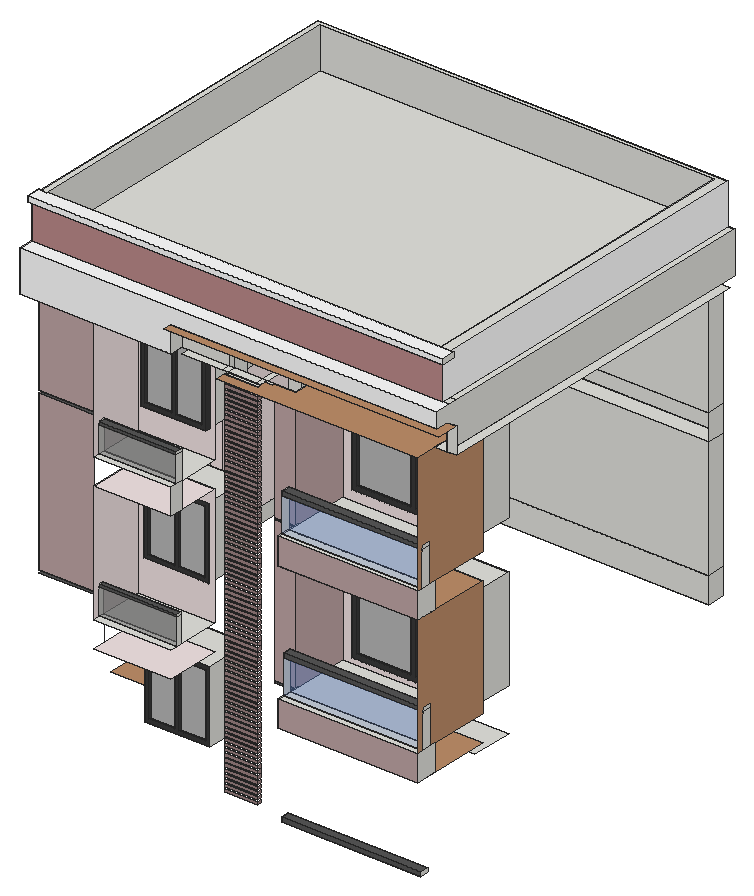
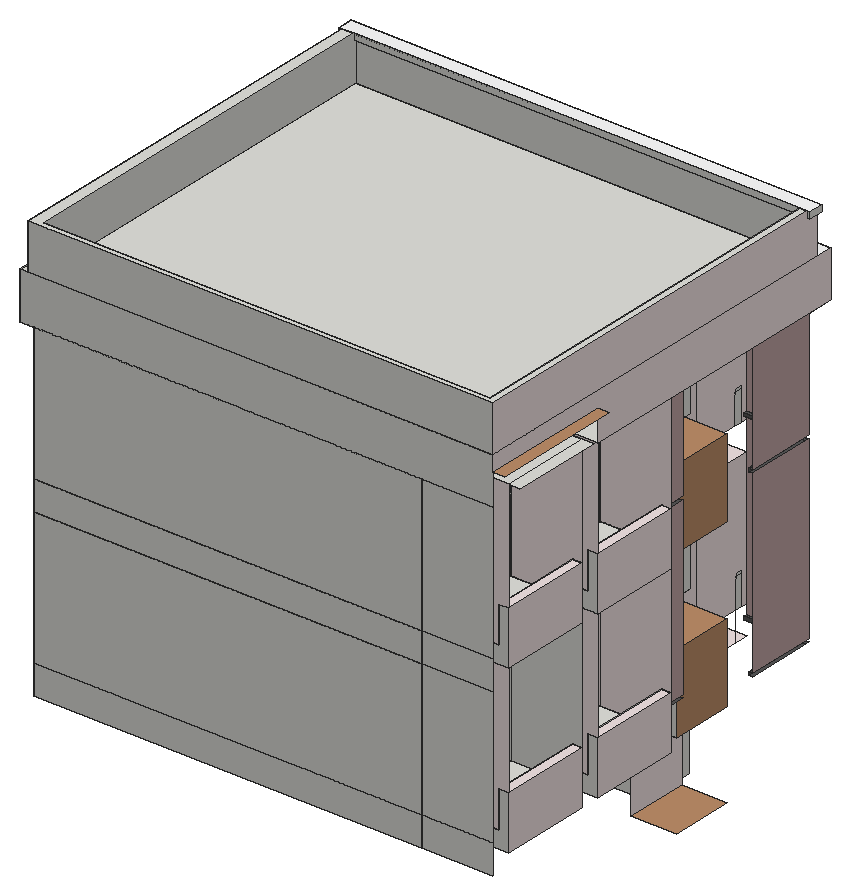
# SketchUp Ruby script. Lengths in inches.
U = 1.inch
M = Sketchup.active_model
def pt(a) = Geom::Point3d.new(a.map { |v| v * U })
def face(e, loops, mat)
  f = e.add_face(loops[0].map { |a| pt(a) })
  loops[1..].each { |l| e.add_face(l.map { |a| pt(a) }).erase! }
  f.material = f.back_material = mat if mat
  f
end
# faces: each face lists its corners as indices into pts; further lists are holes
def faces(e, pts, list, mat = nil) = list.each { |f| face(e, (f[0].is_a?(Array) ? f : [f]).map { |l| l.map { |i| pts[i] } }, mat) }
# xy, xz, yz: faces in a plane at the given z, y or x. An outline is a flat list of corners, or four numbers for a rectangle; further outlines are holes
def ring(l) = l.size == 4 ? [[l[0], l[1]], [l[2], l[1]], [l[2], l[3]], [l[0], l[3]]] : l.each_slice(2).to_a
def flat(e, list, mat, &to3) = list.each { |f| face(e, (f[0].is_a?(Array) ? f : [f]).map { |l| ring(l).map { |u, v| to3.(u, v) } }, mat) }
def xy(e, z, list, mat = nil) = flat(e, list, mat) { |x, y| [x, y, z] }
def xz(e, y, list, mat = nil) = flat(e, list, mat) { |x, z| [x, y, z] }
def yz(e, x, list, mat = nil) = flat(e, list, mat) { |y, z| [x, y, z] }
def lines(e, pts, list) = list.each { |a, b| e.add_line(pt(pts[a]), pt(pts[b])) }
# prism: a flat outline (further loops are holes) pulled along v
def prism(e, loops, v, mat = nil)
  f = face(e, loops, mat); d = Geom::Vector3d.new(v.map { |x| x * U })
  f.pushpull(f.normal.samedirection?(d) ? d.length : -d.length)
end
def box(e, o, s, mat = nil) = prism(e, [[o, [o[0] + s[0], o[1], o[2]], [o[0] + s[0], o[1] + s[1], o[2]], [o[0], o[1] + s[1], o[2]]]], [0, 0, s[2]], mat)
def at(x, y, z, deg = 0) = Geom::Transformation.translation(pt([x, y, z])) * Geom::Transformation.rotation(ORIGIN, Z_AXIS, deg.degrees)
def axes(o, x, y, z) = Geom::Transformation.new([*x, 0, *y, 0, *z, 0, *pt(o).to_a, 1])
def part(name) = M.definitions.add(name)
# library, detail: a bought-in or finely detailed component or shape, given as its bounding box
def library(name, o, s) = part(name).tap { |d| box(d.entities, o, s) }
def detail(e, o, s) = box(e.add_group.entities, o, s)
def put(e, d, t, mat = nil) = e.add_instance(d, t).tap { |i| i.material = mat if mat }
def group(e, t, mat = nil) = e.add_group.tap { |g| g.transformation = t; g.material = mat if mat }.entities
root = M.entities
M.materials.add("Generic").color = [188, 139, 139]
M.materials.add("Generic\#1").color = [192, 166, 166]
M.materials.add("Generic\#2").color = [190, 142, 105]
M.materials.add("Generic\#3").color = [158, 131, 131]
M.materials.add("Generic\#4").color = [242, 228, 228]
M.materials.add("[Color M00]").color = [255, 255, 255]
M.materials.add("[Color M06]").color = [86, 86, 86]
M.materials.add("[Color M07]").color = [58, 58, 58]
M.materials.add("[Mirror 01]").color = [183, 183, 183]
M.materials.add("[Translucent Glass Blue]").color = [98, 147, 234]
M.materials["[Translucent Glass Blue]"].alpha = 0.21
M.materials.add("[Translucent Glass Gray]").color = [128, 128, 128]
M.materials["[Translucent Glass Gray]"].alpha = 0.5
c1 = part("Group\#1")
xy(c1.entities,0,[[0,0,90.75,6]],"[Color M07]")
xy(c1.entities,5.41,[[5.41,0,42.67,3],[48.08,0,85.34,3]],"[Color M07]")
xy(c1.entities,95.34,[[5.41,0,42.67,3],[48.08,0,85.34,3]],"[Color M07]")
xy(c1.entities,100.75,[[0,0,90.75,6]],"[Color M07]")
xz(c1.entities,0,[[[0,0,90.75,100.75],[48.08,5.41,85.34,95.34],[5.41,5.41,42.67,95.34]]],"[Color M07]")
xz(c1.entities,3,[[5.41,5.41,42.67,95.34],[48.08,5.41,85.34,95.34]],"[Mirror 01]")
xz(c1.entities,6,[[0,0,90.75,100.75]],"[Mirror 01]")
yz(c1.entities,0,[[0,0,6,100.75]],"[Color M07]")
yz(c1.entities,5.41,[[0,5.41,3,95.34]],"[Color M07]")
yz(c1.entities,42.67,[[0,5.41,3,95.34]],"[Color M07]")
yz(c1.entities,48.08,[[0,5.41,3,95.34]],"[Color M07]")
yz(c1.entities,85.34,[[0,5.41,3,95.34]],"[Color M07]")
yz(c1.entities,90.75,[[0,0,6,100.75]],"[Color M07]")
c2 = part("Group\#3")
xy(c2.entities,0,[[0,0,45.875,5.125]])
xz(c2.entities,0,[[0,0,45.875,4.1875]])
yz(c2.entities,45.875,[[0,0,5.125,4.1875]])
c3 = part("Group\#2")
xy(c3.entities,0,[[0,0,173,6]],"[Color M07]")
xy(c3.entities,7.67,[[90.33,0,165.33,3]],"[Color M06]")
xy(c3.entities,7.67,[[7.67,0,82.67,3]],"[Color M07]")
xy(c3.entities,134.58,[[7.67,0,82.67,3],[90.33,0,165.33,3]],"[Color M07]")
xy(c3.entities,142.25,[[0,0,173,6]],"[Color M07]")
xz(c3.entities,0,[[[0,0,173,142.25],[7.67,7.67,82.67,134.58],[90.33,7.67,165.33,134.58]]],"[Color M07]")
xz(c3.entities,3,[[7.67,7.67,82.67,134.58],[90.33,7.67,165.33,134.58]],"[Mirror 01]")
xz(c3.entities,6,[[0,0,173,142.25]],"[Mirror 01]")
yz(c3.entities,0,[[0,0,6,142.25]],"[Color M07]")
yz(c3.entities,7.67,[[0,7.67,3,134.58]],"[Color M07]")
yz(c3.entities,82.67,[[0,7.67,3,134.58]],"[Color M07]")
yz(c3.entities,90.33,[[0,7.67,3,134.58]],"[Color M07]")
yz(c3.entities,165.33,[[0,7.67,3,134.58]],"[Color M07]")
yz(c3.entities,173,[[0,0,6,142.25]],"[Color M07]")
xy(root,455.21,[[162.5,105,253.25,171.75]])
xy(root,457.125,[[421.3125,20.9,617.3125,32.9]])
xy(root,462.9375,[[421.3125,20.9,617.3125,32.9]],"[Color M06]")
xy(root,470.25,[[80.75,147.9375,137.3125,225.85]],"Generic\#2")
xy(root,555.96,[[162.5,105,253.25,171.75]])
xy(root,559.68,[[434.09,128.4375,607.09,187.0625]])
xy(root,577.125,[[137.3125,525.6875,145.6875,549.6875],[145.6875,525.6875,617.3125,549.6875]])
xy(root,577.125,[[421.3125,15.0625,617.3125,128.4375],[80.75,147.9375,137.3125,225.85]],"Generic\#2")
xy(root,577.125,[[152.75,27.5625,261.3125,105]],"Generic\#4")
xy(root,592.1875,[[49.25,273.85,137.3125,387.77],[49.25,411.77,137.3125,525.6875]],"Generic\#4")
xy(root,610.6875,[[392.6875,45.6875,421.3125,50.375]],"[Color M06]")
xy(root,613.6875,[[421.3125,15.0625,617.3125,24.5],[421.3125,24.5,617.3125,36.5],[152.75,27.5625,261.3125,37.125],[421.3125,36.5,617.3125,128.4375],[152.75,37.125,261.3125,44.125],
  [152.75,44.125,261.3125,105],[61.25,273.85,137.3125,387.77],[61.25,411.77,137.3125,525.6875],[137.3125,525.6875,145.6875,549.6875],[145.6875,525.6875,617.3125,549.6875]])
xy(root,613.6875,[[392.6875,45.6875,421.3125,50.375]],"[Color M06]")
xy(root,620.55,[[434.09,128.4375,607.09,187.0625]])
xy(root,621.63,[[49.25,61.3125,126.1875,66],[49.25,66,53.9375,147.9375]],"[Color M06]")
xy(root,623.77,[[73.1875,225.85,77.875,249.85]],"[Color M06]")
xy(root,625.63,[[49.25,61.3125,126.1875,66],[49.25,66,53.9375,147.9375]],"[Color M06]")
xy(root,627.77,[[73.1875,225.85,77.875,249.85]],"[Color M06]")
xy(root,650.625,[[152.75,37.125,261.3125,44.125]])
xy(root,654.1875,[[152.75,37.125,261.3125,44.125]],"[Color M06]")
xy(root,658.8125,[[49.25,273.85,61.25,387.77],[49.25,411.77,61.25,525.6875]],"Generic\#4")
xy(root,660.15,[[161.5625,105,252.3125,171.75]])
xy(root,661.6875,[[421.3125,24.5,617.3125,36.5]])
xy(root,667.5,[[421.3125,24.5,617.3125,36.5]],"[Color M06]")
xy(root,674.8125,[[80.75,147.9375,137.3125,225.85]],"Generic\#2")
xy(root,760.9,[[161.5625,105,252.3125,171.75]])
xy(root,762.8,[[434.09,128.4375,607.09,187.0625]])
xy(root,781.6875,[[137.3125,525.6875,617.3125,549.6875]])
xy(root,781.6875,[[421.3125,15.0625,617.3125,128.4375],[80.75,147.9375,137.3125,225.85]],"Generic\#2")
xy(root,781.6875,[[152.75,27.5625,261.3125,105]],"Generic\#4")
xy(root,796.75,[[49.25,273.85,137.3125,387.77],[49.25,411.77,137.3125,525.6875]],"Generic\#4")
xy(root,815.25,[[392.6875,45.6875,421.3125,50.375]],"[Color M06]")
xy(root,818.25,[[421.3125,15.0625,617.3125,22.5625],[421.3125,22.5625,617.3125,34.5625],[152.75,27.5625,261.3125,36.375],[421.3125,34.5625,617.3125,128.4375],[152.75,36.375,261.3125,45.6875],
  [152.75,45.6875,261.3125,105],[61.25,273.85,137.3125,387.77],[61.25,411.77,137.3125,525.6875],[137.3125,525.6875,617.3125,549.6875]])
xy(root,818.25,[[392.6875,45.6875,421.3125,50.375]],"[Color M06]")
xy(root,831.74,[[434.09,128.4375,607.09,187.0625]])
xy(root,843.44,[[73.1875,225.85,77.875,249.85]],"[Color M06]")
xy(root,847.32,[[49.25,61.3125,126.1875,66],[49.25,66,53.9375,147.9375]],"[Color M06]")
xy(root,847.44,[[73.1875,225.85,77.875,249.85]],"[Color M06]")
xy(root,851.32,[[49.25,61.3125,126.1875,66],[49.25,66,53.9375,147.9375]],"[Color M06]")
xy(root,854.96,[[161.8125,105,252.5625,171.75]])
xy(root,855.1875,[[152.75,36.375,261.3125,45.6875]])
xy(root,858.75,[[152.75,36.375,261.3125,45.6875]],"[Color M06]")
xy(root,863.375,[[49.25,273.85,61.25,387.77],[49.25,411.77,61.25,525.6875]],"Generic\#4")
xy(root,866.25,[[421.3125,22.5625,617.3125,34.5625]])
xy(root,872.0625,[[421.3125,22.5625,617.3125,34.5625]],"[Color M06]")
xy(root,879.375,[[80.75,147.9375,137.3125,225.85]],"Generic\#2")
xy(root,955.71,[[161.8125,105,252.5625,171.75]])
xy(root,973.99,[[434.09,128.4375,607.09,187.0625]])
xy(root,986.25,[[49.25,27.5625,126.1875,61.3125],[126.1875,27.5625,152.75,45.6875],[152.75,27.5625,261.3125,105],[336,28.6875,381.875,33.8125],[271.74,33.8125,328.375,45.6875],
  [328.375,33.8125,336,45.6875],[336,33.8125,375.18,45.6875],[375.18,33.8125,381.875,45.6875],[381.875,41.875,392.6875,45.6875],[375.18,45.6875,381.875,157.1],
  [617.3125,45.6875,634.3125,128.4375],[634.3125,45.6875,647.125,525.6875],[617.3125,128.4375,634.3125,525.6875],[49.25,147.9375,49.25,249.85,73.1875,249.85,73.1875,225.85,137.3125,225.85,137.3125,147.9375],[73.1875,225.85,137.3125,249.85],
  [49.25,249.85,137.3125,273.85],[49.25,273.85,137.3125,387.77],[137.3125,525.6875,617.3125,549.6875],[617.3125,525.6875,634.3125,549.6875]])
xy(root,986.25,[[336,15.0625,336,28.6875,381.875,28.6875,381.875,41.875,392.6875,41.875,392.6875,45.6875,421.3125,45.6875,421.3125,128.4375,617.3125,128.4375,617.3125,15.0625]],"Generic\#2")
xy(root,1000.9375,[[34.875,411.77,49.25,525.6875],[49.25,411.77,137.3125,525.6875]])
xy(root,1022.8125,[[261.3125,27.5625,634.3125,45.6875]])
xy(root,1022.8125,[[261.3125,15.0625,647.125,15.0625,647.125,45.6875,634.3125,45.6875,634.3125,27.5625,261.3125,27.5625]],"Generic\#2")
xy(root,1024.8125,[[34.875,387.77,49.25,549.6875]],"Generic\#2")
xy(root,1044.4375,[[[49.25,48.6875,624.9375,549.6875],[58.0625,60.6875,609.9375,543.0625]],[624.9375,48.6875,634.3125,60.6875],[58.0625,60.6875,609.9375,543.0625],[624.9375,60.6875,634.3125,549.6875]])
xy(root,1044.4375,[[49.25,27.5625,634.3125,48.6875]],"[Color M00]")
xy(root,1093.625,[[45.75,45.1875,628.4375,48.6875],[45.75,48.6875,49.25,64.1875],[49.25,48.6875,49.25,64.1875,58.0625,64.1875,58.0625,60.6875,624.9375,60.6875,624.9375,48.6875],[624.9375,48.6875,628.4375,60.6875],[58.0625,60.6875,609.9375,64.1875],
  [609.9375,60.6875,624.9375,64.1875],[624.9375,60.6875,628.4375,64.1875]])
xy(root,1101.375,[[49.25,64.1875,58.0625,64.1875,58.0625,543.0625,609.9375,543.0625,609.9375,64.1875,624.9375,64.1875,624.9375,549.6875,49.25,549.6875]])
xy(root,1101.375,[[45.75,45.1875,628.4375,64.1875]],"[Color M00]")
xz(root,15.0625,[[421.3125,577.125,617.3125,613.6875],[421.3125,781.6875,617.3125,818.25]],"Generic\#1")
xz(root,20.9,[[421.3125,457.125,617.3125,462.9375]],"[Color M06]")
xz(root,22.5625,[[421.3125,866.25,617.3125,872.0625]],"[Color M06]")
xz(root,22.5625,[[421.3125,818.25,617.3125,866.25]],"[Translucent Glass Blue]")
xz(root,24.5,[[421.3125,661.6875,617.3125,667.5]],"[Color M06]")
xz(root,24.5,[[421.3125,613.6875,617.3125,661.6875]],"[Translucent Glass Blue]")
xz(root,27.5625,[[49.25,986.25,261.3125,986.25,261.3125,1022.8125,634.3125,1022.8125,634.3125,1044.4375,49.25,1044.4375]],"[Color M00]")
xz(root,32.9,[[421.3125,457.125,617.3125,462.9375]])
xz(root,33.8125,[[336,982.0625,375.18,986.25],[375.18,982.0625,381.875,986.25]])
xz(root,34.5625,[[421.3125,866.25,617.3125,872.0625]])
xz(root,34.5625,[[421.3125,818.25,617.3125,866.25]],"[Translucent Glass Blue]")
xz(root,36.375,[[152.75,855.1875,261.3125,858.75]],"[Color M06]")
xz(root,36.375,[[152.75,818.25,261.3125,855.1875]],"[Translucent Glass Gray]")
xz(root,36.5,[[421.3125,661.6875,617.3125,667.5]])
xz(root,36.5,[[421.3125,613.6875,617.3125,661.6875]],"[Translucent Glass Blue]")
xz(root,37.125,[[152.75,650.625,261.3125,654.1875]],"[Color M06]")
xz(root,37.125,[[152.75,613.6875,261.3125,650.625]],"[Translucent Glass Gray]")
xz(root,44.125,[[152.75,650.625,261.3125,654.1875]])
xz(root,44.125,[[152.75,613.6875,261.3125,650.625]],"[Translucent Glass Gray]")
xz(root,45.1875,[[45.75,1093.625,628.4375,1101.375]],"[Color M00]")
xz(root,45.6875,[[152.75,855.1875,261.3125,858.75],[261.3125,986.25,328.375,1022.8125],[634.3125,986.25,647.125,1022.8125]])
xz(root,45.6875,[[392.6875,613.6875,421.3125,815.25],[392.6875,818.25,421.3125,986.25]],"Generic\#1")
xz(root,45.6875,[[152.75,818.25,261.3125,855.1875]],"[Translucent Glass Gray]")
xz(root,48.6875,[[49.25,1044.4375,624.9375,1093.625]],"Generic")
xz(root,50.375,[[392.6875,610.6875,421.3125,613.6875],[392.6875,815.25,421.3125,818.25]],"[Color M06]")
xz(root,60.6875,[[58.0625,1044.4375,609.9375,1093.625]])
xz(root,61.3125,[[49.25,625.63,126.1875,847.32],[49.25,851.32,126.1875,986.25]],"Generic\#1")
xz(root,64.1875,[[45.75,1093.625,49.25,1101.375],[49.25,1093.625,58.0625,1101.375],[58.0625,1093.625,609.9375,1101.375],[609.9375,1093.625,624.9375,1101.375],[624.9375,1093.625,628.4375,1101.375]])
xz(root,66,[[53.9375,621.63,126.1875,625.63],[53.9375,847.32,126.1875,851.32]],"[Color M06]")
xz(root,105,[[[152.75,613.6875,261.3125,781.6875],[161.5625,660.15,252.3125,760.9]],[[152.75,818.25,261.3125,986.25],[161.8125,854.96,252.5625,955.71]]],"Generic\#4")
xz(root,128.4375,[[[421.3125,613.6875,617.3125,781.6875],[434.09,620.55,607.09,762.8]],[[421.3125,818.25,617.3125,986.25],[434.09,831.74,607.09,973.99]]],"Generic\#4")
xz(root,171.75,[[162.5,455.21,253.25,555.96],[161.5625,660.15,252.3125,760.9],[161.8125,854.96,252.5625,955.71]])
xz(root,187.0625,[[434.09,620.55,607.09,762.8],[434.09,831.74,607.09,973.99]])
xz(root,225.85,[[80.75,577.125,137.3125,674.8125],[80.75,781.6875,137.3125,879.375]])
xz(root,249.85,[[73.1875,577.125,137.3125,613.6875],[73.1875,613.6875,137.3125,613.6875,137.3125,781.6875,73.1875,781.6875,73.1875,627.77,77.875,627.77,77.875,623.77,73.1875,623.77],[73.1875,781.6875,137.3125,818.25],[73.1875,818.25,137.3125,818.25,137.3125,986.25,73.1875,986.25,73.1875,847.44,77.875,847.44,77.875,843.44,73.1875,843.44]])
xz(root,273.85,[[49.25,592.1875,49.25,658.8125,61.25,658.8125,61.25,613.6875,137.3125,613.6875,137.3125,592.1875],[49.25,796.75,49.25,863.375,61.25,863.375,61.25,818.25,137.3125,818.25,137.3125,796.75]])
xz(root,273.85,[[61.25,613.6875,61.25,658.8125,49.25,658.8125,49.25,796.75,137.3125,796.75,137.3125,613.6875],[61.25,818.25,61.25,863.375,49.25,863.375,49.25,986.25,137.3125,986.25,137.3125,818.25]],"Generic\#4")
xz(root,387.77,[[49.25,592.1875,137.3125,592.1875,137.3125,613.6875,61.25,613.6875,61.25,658.8125,49.25,658.8125],[49.25,796.75,137.3125,796.75,137.3125,818.25,61.25,818.25,61.25,863.375,49.25,863.375]])
xz(root,387.77,[[61.25,613.6875,137.3125,613.6875,137.3125,796.75,49.25,796.75,49.25,658.8125,61.25,658.8125],[61.25,818.25,137.3125,818.25,137.3125,986.25,49.25,986.25,49.25,863.375,61.25,863.375]],"Generic\#4")
xz(root,411.77,[[49.25,592.1875,49.25,658.8125,61.25,658.8125,61.25,613.6875,137.3125,613.6875,137.3125,592.1875],[61.25,613.6875,61.25,658.8125,49.25,658.8125,49.25,796.75,137.3125,796.75,137.3125,613.6875],[49.25,796.75,49.25,863.375,61.25,863.375,61.25,818.25,137.3125,818.25,137.3125,796.75]])
xz(root,411.77,[[61.25,818.25,61.25,863.375,49.25,863.375,49.25,1000.9375,137.3125,1000.9375,137.3125,818.25]],"Generic\#4")
xz(root,525.6875,[[137.3125,577.125,145.6875,613.6875],[145.6875,577.125,617.3125,613.6875],[49.25,592.1875,137.3125,592.1875,137.3125,613.6875,61.25,613.6875,61.25,658.8125,49.25,658.8125],[137.3125,613.6875,617.3125,781.6875],[49.25,796.75,137.3125,796.75,137.3125,818.25,61.25,818.25,61.25,863.375,49.25,863.375],
  [137.3125,818.25,617.3125,986.25]])
xz(root,525.6875,[[61.25,613.6875,137.3125,613.6875,137.3125,796.75,49.25,796.75,49.25,658.8125,61.25,658.8125],[61.25,818.25,137.3125,818.25,137.3125,1000.9375,49.25,1000.9375,49.25,863.375,61.25,863.375]],"Generic\#4")
xz(root,543.0625,[[58.0625,1044.4375,609.9375,1101.375]])
xz(root,549.6875,[[49.25,577.125,137.3125,613.6875],[137.3125,577.125,617.3125,613.6875],[49.25,613.6875,137.3125,781.6875],[137.3125,613.6875,617.3125,781.6875],[49.25,781.6875,137.3125,818.25],
  [137.3125,781.6875,617.3125,818.25],[49.25,818.25,137.3125,986.25],[137.3125,818.25,617.3125,986.25],[49.25,986.25,634.3125,1044.4375],[49.25,1044.4375,624.9375,1101.375]])
yz(root,45.75,[[45.1875,1093.625,64.1875,1101.375]])
yz(root,49.25,[[61.3125,625.63,147.9375,847.32],[61.3125,851.32,147.9375,986.25]],"Generic\#1")
yz(root,49.25,[[273.85,592.1875,387.77,658.8125],[411.77,592.1875,525.6875,658.8125],[273.85,796.75,387.77,863.375],[411.77,796.75,525.6875,863.375],[27.5625,986.25,27.5625,1044.4375,549.6875,1044.4375,549.6875,1024.8125,387.77,1024.8125,387.77,986.25],
  [48.6875,1044.4375,48.6875,1093.625,64.1875,1093.625,64.1875,1101.375,549.6875,1101.375,549.6875,1044.4375]],"Generic\#4")
yz(root,53.9375,[[66,621.63,147.9375,625.63],[66,847.32,147.9375,851.32]],"[Color M06]")
yz(root,58.0625,[[60.6875,1044.4375,543.0625,1044.4375,543.0625,1101.375,64.1875,1101.375,64.1875,1093.625,60.6875,1093.625]])
yz(root,61.25,[[273.85,613.6875,387.77,658.8125],[411.77,613.6875,525.6875,658.8125],[273.85,818.25,387.77,863.375],[411.77,818.25,525.6875,863.375]])
yz(root,73.1875,[[225.85,627.77,249.85,843.44],[225.85,847.44,249.85,986.25]],"Generic\#1")
yz(root,77.875,[[225.85,623.77,249.85,627.77],[225.85,843.44,249.85,847.44]],"[Color M06]")
yz(root,80.75,[[147.9375,577.125,225.85,674.8125],[147.9375,781.6875,225.85,879.375]],"Generic\#2")
yz(root,137.3125,[[157.1,577.125,225.85,674.8125],[525.6875,577.125,549.6875,613.6875],[273.85,592.1875,387.77,613.6875],[411.77,592.1875,525.6875,613.6875],[411.77,613.6875,525.6875,796.75],
  [525.6875,613.6875,549.6875,781.6875],[157.1,781.6875,225.85,796.75],[525.6875,781.6875,549.6875,818.25],[157.1,796.75,225.85,879.375],[225.85,796.75,249.85,986.25],
  [249.85,796.75,273.85,986.25],[273.85,796.75,387.77,818.25],[387.77,796.75,411.77,986.25],[411.77,796.75,525.6875,818.25],[273.85,818.25,387.77,986.25],
  [411.77,818.25,525.6875,986.25],[525.6875,818.25,549.6875,986.25]])
yz(root,137.3125,[[147.9375,470.25,225.85,577.125],[273.85,613.6875,387.77,796.75],[147.9375,674.8125,225.85,781.6875],[147.9375,879.375,225.85,986.25],[411.77,986.25,525.6875,1000.9375]],"Generic\#4")
yz(root,152.75,[[37.125,613.6875,44.125,650.625],[37.125,650.625,44.125,654.1875],[36.375,818.25,45.6875,855.1875],[36.375,855.1875,45.6875,858.75]])
yz(root,152.75,[[27.5625,613.6875,37.125,613.6875,37.125,654.1875,44.125,654.1875,44.125,613.6875,105,613.6875,105,781.6875,27.5625,781.6875],[27.5625,818.25,36.375,818.25,36.375,858.75,45.6875,858.75,45.6875,818.25,105,818.25,105,986.25,27.5625,986.25]],"Generic\#4")
yz(root,161.5625,[[105,660.15,171.75,760.9]])
yz(root,161.8125,[[105,854.96,171.75,955.71]])
yz(root,162.5,[[105,455.21,171.75,555.96]])
yz(root,252.3125,[[105,660.15,171.75,760.9]])
yz(root,252.5625,[[105,854.96,171.75,955.71]])
yz(root,253.25,[[105,455.21,171.75,555.96]])
yz(root,261.3125,[[37.125,613.6875,44.125,650.625],[37.125,650.625,44.125,654.1875],[27.5625,781.6875,45.6875,818.25],[36.375,818.25,45.6875,855.1875],[36.375,855.1875,45.6875,858.75],
  [27.5625,986.25,45.6875,1022.8125]])
yz(root,336,[[28.6875,982.0625,33.8125,986.25]])
yz(root,392.6875,[[45.6875,610.6875,50.375,613.6875],[45.6875,815.25,50.375,818.25]],"[Color M06]")
yz(root,421.3125,[[20.9,457.125,32.9,462.9375],[15.0625,577.125,15.0625,613.6875,50.375,613.6875,50.375,610.6875,45.6875,610.6875,45.6875,577.125],[24.5,613.6875,36.5,661.6875],[24.5,661.6875,36.5,667.5],[15.0625,781.6875,15.0625,818.25,50.375,818.25,50.375,815.25,45.6875,815.25,45.6875,781.6875],
  [22.5625,818.25,34.5625,866.25],[22.5625,866.25,34.5625,872.0625]])
yz(root,421.3125,[[45.6875,613.6875,128.4375,781.6875],[45.6875,818.25,128.4375,986.25]],"Generic\#1")
yz(root,434.09,[[128.4375,620.55,187.0625,762.8],[128.4375,831.74,187.0625,973.99]])
yz(root,607.09,[[128.4375,620.55,187.0625,762.8],[128.4375,831.74,187.0625,973.99]])
yz(root,609.9375,[[60.6875,1044.4375,60.6875,1093.625,64.1875,1093.625,64.1875,1101.375,543.0625,1101.375,543.0625,1044.4375]])
yz(root,617.3125,[[20.9,457.125,32.9,462.9375],[15.0625,577.125,45.6875,613.6875],[525.6875,577.125,549.6875,613.6875],[24.5,613.6875,36.5,661.6875],[525.6875,613.6875,549.6875,781.6875],
  [24.5,661.6875,36.5,667.5],[15.0625,781.6875,45.6875,818.25],[525.6875,781.6875,549.6875,818.25],[22.5625,818.25,34.5625,866.25],[525.6875,818.25,549.6875,986.25],
  [22.5625,866.25,34.5625,872.0625]])
yz(root,617.3125,[[15.0625,613.6875,15.0625,781.6875,128.4375,781.6875,128.4375,613.6875,36.5,613.6875,36.5,667.5,24.5,667.5,24.5,613.6875],[15.0625,818.25,15.0625,986.25,128.4375,986.25,128.4375,818.25,34.5625,818.25,34.5625,872.0625,22.5625,872.0625,22.5625,818.25]],"Generic\#2")
yz(root,624.9375,[[48.6875,1044.4375,549.6875,1044.4375,549.6875,1101.375,64.1875,1101.375,64.1875,1093.625,48.6875,1093.625]],"[Color M00]")
yz(root,628.4375,[[45.1875,1093.625,64.1875,1101.375]])
yz(root,634.3125,[[45.6875,986.25,549.6875,986.25,549.6875,1044.4375,27.5625,1044.4375,27.5625,1022.8125,45.6875,1022.8125]])
p = [[336,45.6875,986.25],[336,45.6875,1022.8125],[152.75,45.6875,613.6875],[152.75,45.6875,577.125],[271.74,157.1,986.25],[137.3125,157.1,986.25]]
lines(root,p,[[0,1],[2,3],[4,5]])
put(root,c1,at(162.5,105,455.21))
put(root,c2,at(336,28.6875,460.625),"Generic\#3")
put(root,c2,at(336,28.6875,467.0625),"Generic\#3")
put(root,c2,at(336,28.6875,473.5),"Generic\#3")
put(root,c2,at(336,28.6875,479.9375),"Generic\#3")
put(root,c2,at(336,28.6875,486.375),"Generic\#3")
put(root,c2,at(336,28.6875,492.8125),"Generic\#3")
put(root,c2,at(336,28.6875,499.25),"Generic\#3")
put(root,c2,at(336,28.6875,505.6875),"Generic\#3")
put(root,c2,at(336,28.6875,512.125),"Generic\#3")
put(root,c2,at(336,28.6875,518.5625),"Generic\#3")
put(root,c2,at(336,28.6875,525),"Generic\#3")
put(root,c2,at(336,28.6875,531.4375),"Generic\#3")
put(root,c2,at(336,28.6875,537.875),"Generic\#3")
put(root,c2,at(336,28.6875,544.3125),"Generic\#3")
put(root,c2,at(336,28.6875,550.75),"Generic\#3")
put(root,c2,at(336,28.6875,557.1875),"Generic\#3")
put(root,c2,at(336,28.6875,563.625),"Generic\#3")
put(root,c2,at(336,28.6875,570.0625),"Generic\#3")
put(root,c2,at(336,28.6875,576.5),"Generic\#3")
put(root,c2,at(336,28.6875,582.9375),"Generic\#3")
put(root,c2,at(336,28.6875,589.375),"Generic\#3")
put(root,c2,at(336,28.6875,595.8125),"Generic\#3")
put(root,c2,at(336,28.6875,602.25),"Generic\#3")
put(root,c2,at(336,28.6875,608.6875),"Generic\#3")
put(root,c2,at(336,28.6875,615.125),"Generic\#3")
put(root,c3,at(434.09,128.4375,620.55))
put(root,c2,at(336,28.6875,621.5625),"Generic\#3")
put(root,c2,at(336,28.6875,628),"Generic\#3")
put(root,c2,at(336,28.6875,634.4375),"Generic\#3")
put(root,c2,at(336,28.6875,640.875),"Generic\#3")
put(root,c2,at(336,28.6875,647.3125),"Generic\#3")
put(root,c2,at(336,28.6875,653.75),"Generic\#3")
put(root,c1,at(161.5625,105,660.15),"Generic\#4")
put(root,c2,at(336,28.6875,660.1875),"Generic\#3")
put(root,c2,at(336,28.6875,666.625),"Generic\#3")
put(root,c2,at(336,28.6875,673.0625),"Generic\#3")
put(root,c2,at(336,28.6875,679.5),"Generic\#3")
put(root,c2,at(336,28.6875,685.9375),"Generic\#3")
put(root,c2,at(336,28.6875,692.375),"Generic\#3")
put(root,c2,at(336,28.6875,698.8125),"Generic\#3")
put(root,c2,at(336,28.6875,705.25),"Generic\#3")
put(root,c2,at(336,28.6875,711.6875),"Generic\#3")
put(root,c2,at(336,28.6875,718.125),"Generic\#3")
put(root,c2,at(336,28.6875,724.5625),"Generic\#3")
put(root,c2,at(336,28.6875,731),"Generic\#3")
put(root,c2,at(336,28.6875,737.4375),"Generic\#3")
put(root,c2,at(336,28.6875,743.875),"Generic\#3")
put(root,c2,at(336,28.6875,750.3125),"Generic\#3")
put(root,c2,at(336,28.6875,756.75),"Generic\#3")
put(root,c2,at(336,28.6875,763.1875),"Generic\#3")
put(root,c2,at(336,28.6875,769.625),"Generic\#3")
put(root,c2,at(336,28.6875,776.0625),"Generic\#3")
put(root,c2,at(336,28.6875,782.5),"Generic\#3")
put(root,c2,at(336,28.6875,788.9375),"Generic\#3")
put(root,c2,at(336,28.6875,795.375),"Generic\#3")
put(root,c2,at(336,28.6875,801.8125),"Generic\#3")
put(root,c2,at(336,28.6875,808.25),"Generic\#3")
put(root,c2,at(336,28.6875,814.6875),"Generic\#3")
put(root,c2,at(336,28.6875,821.125),"Generic\#3")
put(root,c2,at(336,28.6875,827.5625),"Generic\#3")
put(root,c3,at(434.09,128.4375,831.74))
put(root,c2,at(336,28.6875,834),"Generic\#3")
put(root,c2,at(336,28.6875,840.4375),"Generic\#3")
put(root,c2,at(336,28.6875,846.875),"Generic\#3")
put(root,c2,at(336,28.6875,853.3125),"Generic\#3")
put(root,c1,at(162.25,99,854.96))
put(root,c2,at(336,28.6875,859.75),"Generic\#3")
put(root,c2,at(336,28.6875,866.1875),"Generic\#3")
put(root,c2,at(336,28.6875,872.625),"Generic\#3")
put(root,c2,at(336,28.6875,879.0625),"Generic\#3")
put(root,c2,at(336,28.6875,885.5),"Generic\#3")
put(root,c2,at(336,28.6875,891.9375),"Generic\#3")
put(root,c2,at(336,28.6875,898.375),"Generic\#3")
put(root,c2,at(336,28.6875,904.8125),"Generic\#3")
put(root,c2,at(336,28.6875,911.25),"Generic\#3")
put(root,c2,at(336,28.6875,917.6875),"Generic\#3")
put(root,c2,at(336,28.6875,924.125),"Generic\#3")
put(root,c2,at(336,28.6875,930.5625),"Generic\#3")
put(root,c2,at(336,28.6875,937),"Generic\#3")
put(root,c2,at(336,28.6875,943.4375),"Generic\#3")
put(root,c2,at(336,28.6875,949.875),"Generic\#3")
put(root,c2,at(336,28.6875,956.3125),"Generic\#3")
put(root,c2,at(336,28.6875,962.75),"Generic\#3")
put(root,c2,at(336,28.6875,969.1875),"Generic\#3")
put(root,c2,at(336,28.6875,975.625),"Generic\#3")
put(root,c2,at(336,28.6875,982.0625),"Generic\#3")
